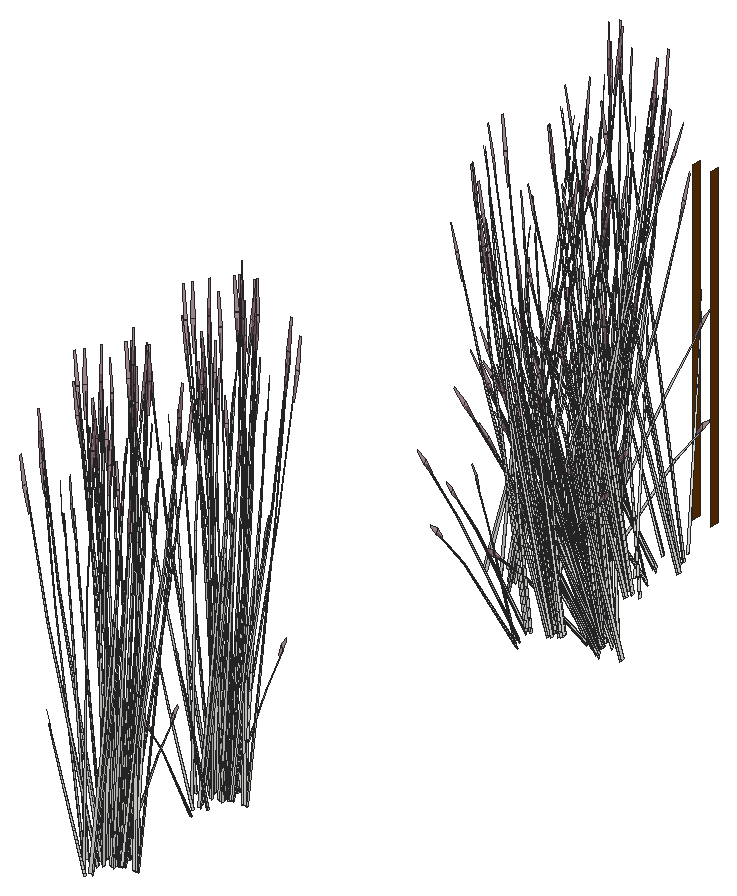
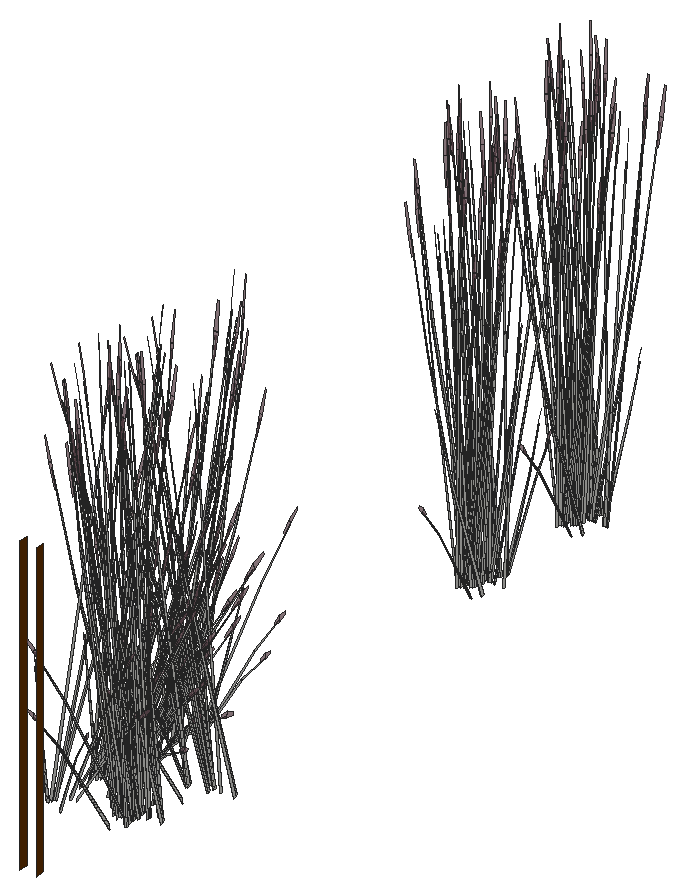
# SketchUp Ruby script. Lengths in inches.
U = 1.inch
M = Sketchup.active_model
def pt(a) = Geom::Point3d.new(a.map { |v| v * U })
def face(e, loops, mat)
  f = e.add_face(loops[0].map { |a| pt(a) })
  loops[1..].each { |l| e.add_face(l.map { |a| pt(a) }).erase! }
  f.material = f.back_material = mat if mat
  f
end
# faces: each face lists its corners as indices into pts; further lists are holes
def faces(e, pts, list, mat = nil) = list.each { |f| face(e, (f[0].is_a?(Array) ? f : [f]).map { |l| l.map { |i| pts[i] } }, mat) }
# xy, xz, yz: faces in a plane at the given z, y or x. An outline is a flat list of corners, or four numbers for a rectangle; further outlines are holes
def ring(l) = l.size == 4 ? [[l[0], l[1]], [l[2], l[1]], [l[2], l[3]], [l[0], l[3]]] : l.each_slice(2).to_a
def flat(e, list, mat, &to3) = list.each { |f| face(e, (f[0].is_a?(Array) ? f : [f]).map { |l| ring(l).map { |u, v| to3.(u, v) } }, mat) }
def xy(e, z, list, mat = nil) = flat(e, list, mat) { |x, y| [x, y, z] }
def xz(e, y, list, mat = nil) = flat(e, list, mat) { |x, z| [x, y, z] }
def yz(e, x, list, mat = nil) = flat(e, list, mat) { |y, z| [x, y, z] }
def lines(e, pts, list) = list.each { |a, b| e.add_line(pt(pts[a]), pt(pts[b])) }
# prism: a flat outline (further loops are holes) pulled along v
def prism(e, loops, v, mat = nil)
  f = face(e, loops, mat); d = Geom::Vector3d.new(v.map { |x| x * U })
  f.pushpull(f.normal.samedirection?(d) ? d.length : -d.length)
end
def box(e, o, s, mat = nil) = prism(e, [[o, [o[0] + s[0], o[1], o[2]], [o[0] + s[0], o[1] + s[1], o[2]], [o[0], o[1] + s[1], o[2]]]], [0, 0, s[2]], mat)
def at(x, y, z, deg = 0) = Geom::Transformation.translation(pt([x, y, z])) * Geom::Transformation.rotation(ORIGIN, Z_AXIS, deg.degrees)
def axes(o, x, y, z) = Geom::Transformation.new([*x, 0, *y, 0, *z, 0, *pt(o).to_a, 1])
def part(name) = M.definitions.add(name)
# library, detail: a bought-in or finely detailed component or shape, given as its bounding box
def library(name, o, s) = part(name).tap { |d| box(d.entities, o, s) }
def detail(e, o, s) = box(e.add_group.entities, o, s)
def put(e, d, t, mat = nil) = e.add_instance(d, t).tap { |i| i.material = mat if mat }
def group(e, t, mat = nil) = e.add_group.tap { |g| g.transformation = t; g.material = mat if mat }.entities
root = M.entities
M.materials.add("C08_Toffee_Ember").color = [102, 51, 0]
M.materials.add("LightPink_Translucent").color = [144, 107, 117]
M.materials["LightPink_Translucent"].alpha = 0.75
c1 = part("blade")
p = [[2.15,0.21,22],[0,0.17,0],[0.09,0.45,0],[2.18,0.31,22],[2.29,0.31,22],[0.38,0.45,0],
  [2.48,0.24,33],[2.49,0.24,33],[2.48,0.22,33]]
faces(c1.entities,p,[[0,1,2,3],[4,5,2,3],[6,3,4,7],[8,0,3,6]])
c2 = part("seeds")
p = [[0.3,-0.1,1.38],[-0.01,-0.03,1.59],[-0.01,-0.03,0.03],[0.14,-0.07,-0.07],[0.29,-0.03,3],[0.15,0.01,3.11]]
faces(c2.entities,p,[[0,1,2,3],[1,0,4,5]],"LightPink_Translucent")
c3 = part("blade with seeds")
put(c3.entities,c1,at(0,0,0))
put(c3.entities,c2,axes([2.4,0.25,30.99],[1.5799,-0.05474,1.17369],[-0.12525,1.92788,0.29478],[-0.07173,-0.02425,1.56792]))
yz(root,671.22,[[360,510,361,546]],"C08_Toffee_Ember")
yz(root,673.24,[[360,510,361,546]],"C08_Toffee_Ember")
put(root,c3,axes([670.66,276.35,511.74],[-0.26718,-0.5855,-0.57963],[0.76964,-0.21087,-0.15213],[-0.02953,-0.19827,1.27944]))
put(root,c3,axes([670.56,274.67,511.97],[-0.40676,-0.57214,0],[0.68052,-0.31907,-0.42834],[0.15499,-0.07267,1.3588]))
put(root,c3,axes([671.45,273.98,511.77],[-0.44958,0.32756,-0.03231],[-0.41194,-0.35875,-0.14649],[-0.029,-0.10165,0.48318]))
put(root,c3,axes([669.09,276.27,511.67],[0,-0.57097,-0.4121],[0.72788,0,0],[0,-0.13004,1.30728]))
put(root,c3,axes([671.11,274.58,511.67],[0.60889,-0.28548,-0.4121],[0.36394,0.51192,0],[0.13868,-0.06502,1.30728]))
put(root,c3,axes([671.07,276.5,511.83],[0.31565,-0.51449,-0.37133],[0.65588,0.24761,0.17871],[0,-0.1186,1.19224]))
put(root,c3,axes([671.36,276.25,512.21],[-0.07581,-0.65151,-0.24149],[0.7896,-0.03939,-0.41502],[0.13904,-0.08678,1.32557]))
put(root,c3,axes([669.4,276.28,511.68],[0.45414,-0.35624,-0.25712],[0.45414,0.35624,0.25712],[0,-0.11474,1.15348]))
put(root,c3,axes([670.99,276.93,512.21],[-0.73268,-0.27244,-0.24149],[0.35279,-0.57501,-0.41502],[-0.02303,-0.14118,1.32557]))
put(root,c3,axes([671.25,274.8,511.68],[0.60696,0.14127,-0.25712],[-0.15283,0.49751,0.25712],[0.12236,-0.05737,1.15348]))
put(root,c3,axes([671.46,276.76,512.02],[0.73304,0.27674,0.19974],[-0.35279,0.57501,0.41502],[0,-0.13255,1.3325]))
put(root,c3,axes([671.2,276.58,511.96],[0.28286,0.63846,0.37976],[-0.80821,0.22202,0.14902],[0.00988,-0.11732,1.31851]))
put(root,c3,axes([672.22,276.64,511.83],[0,-0.66065,0],[0.81352,0,0],[0,0,1.48949]))
put(root,c3,axes([671.83,276.22,511.96],[-0.53943,0.51816,0.37976],[-0.64086,-0.4574,0.14902],[0.13005,-0.05171,1.31851]))
put(root,c3,axes([672.42,277.15,511.91],[-0.60515,-0.49144,-0.05089],[0.60552,-0.49174,0],[-0.02113,-0.01716,1.45724]))
put(root,c3,axes([671.27,277.21,511.96],[0.82229,0.1203,0.37976],[-0.16734,0.67942,0.14902],[-0.12017,-0.06561,1.31851]))
put(root,c3,axes([672.77,276.78,511.83],[0.72788,0,0],[0,0.59111,0],[0,0,1.48078]))
put(root,c3,axes([672.53,276.48,511.98],[-0.82229,-0.1203,0.40835],[0.16734,-0.67942,0.16024],[0.12017,0.06561,1.41775]))
put(root,c3,axes([671.88,278.16,511.83],[-0.21227,-0.49226,0],[0.60616,-0.17239,0],[0,0,1.28128]))
put(root,c3,axes([672.75,277.04,511.84],[0.45414,0.3688,0],[-0.45414,0.3688,0],[0,0,1.40491]))
put(root,c3,axes([671.73,278.38,511.82],[-0.65588,-0.25634,0],[0.31565,-0.53263,0],[0,0,1.35047]))
put(root,c3,axes([672.625,276.9,511.9],[0,0.66033,-0.04679],[-0.81352,0,0],[0,0.02075,1.48875]))
put(root,c3,axes([673.02,276.72,512.17],[0.60616,-0.16651,0.12018],[0.21227,0.47548,-0.34318],[0,0.10465,1.05198]))
put(root,c3,axes([672.47,278.39,511.83],[0.65588,0.25634,0],[-0.31565,0.53263,0],[0,0,1.45212]))
put(root,c3,axes([672.73,278.96,511.82],[-0.40169,-0.57414,-0.04268],[0.68052,-0.31907,0.42834],[-0.16769,0.05466,1.35813]))
put(root,c3,axes([672.59,277.57,512.17],[0.48065,0.34305,0.12018],[-0.40092,0.38703,-0.34318],[-0.1116,0.05232,1.05198]))
put(root,c3,axes([672.24,278.18,511.9],[0.28286,0.65594,-0.0499],[-0.80821,0.22985,0],[0.00988,0.02291,1.42904]))
put(root,c3,axes([672.55,278.89,511.68],[-0.60696,-0.14127,-0.25712],[0.15283,-0.49751,0.25712],[-0.12236,0.05737,1.15348]))
put(root,c3,axes([674.57,277.32,511.83],[-0.81312,-0.00457,-0.0413],[0,-0.63814,0.41452],[-0.02555,0.14527,1.31432]))
put(root,c3,axes([672.8125,276.76,512.21],[0.73268,0.27244,-0.24149],[-0.35279,0.57501,-0.41502],[0.02303,0.14118,1.32557]))
put(root,c3,axes([674.4,277.41,511.68],[-0.45414,0.35624,-0.25712],[-0.45414,-0.35624,0.25712],[0,0.11474,1.15348]))
put(root,c3,axes([672.45,277.44,512.21],[0.07581,0.65151,-0.24149],[-0.7896,0.03939,-0.41502],[-0.13904,0.08678,1.32557]))
put(root,c3,axes([672.73,277.19,511.83],[-0.31565,0.51449,-0.37133],[-0.65588,-0.24761,0.17871],[0,0.1186,1.19224]))
put(root,c3,axes([672.75,278.67,511.93],[0.81449,0.18558,0.25528],[-0.20377,0.66335,-0.30288],[-0.13481,0.08302,1.36855]))
put(root,c3,axes([674.72,277.42,511.67],[0,0.57097,-0.4121],[-0.72788,0,0],[0,0.13004,1.30728]))
put(root,c3,axes([673.25,279.02,511.97],[0.40676,0.57214,0],[-0.68052,0.31907,-0.42834],[-0.15499,0.07267,1.3588]))
put(root,c3,axes([673.11,277.35,511.74],[0.23855,0.52277,-0.57446],[-0.68718,0.18827,-0.15077],[0.02637,0.17702,1.26801]))
put(root,c3,axes([671.11,279.2,511.24],[0.10529,-0.03107,1.46364],[0.63335,0.17101,-0.2236],[0.01852,0.19274,0.24931]))
put(root,c3,axes([669.65,279.28,512.34],[0.59102,-0.10111,0.05401],[0.13587,0.40735,-0.71633],[-0.03747,0.2062,0.64209]))
put(root,c3,axes([672.94,289.54,512.15],[-0.18493,0.11557,1.18691],[-0.55384,-0.20228,-0.25526],[0.10266,-0.25157,0.50747]))
put(root,c3,axes([671.5625,288.91,511.24],[-0.10912,0.02057,1.46364],[-0.60346,-0.23156,-0.2236],[0.01013,-0.19315,0.24931]))
put(root,c3,axes([670.66,291.68,511.74],[-0.26718,-0.5855,-0.57963],[0.76964,-0.21087,-0.15213],[-0.02953,-0.19827,1.27944]))
put(root,c3,axes([670.56,290,511.97],[-0.40676,-0.57214,0],[0.68052,-0.31907,-0.42834],[0.15499,-0.07267,1.3588]))
put(root,c3,axes([671.45,289.3125,511.77],[-0.44958,0.32756,-0.03231],[-0.41194,-0.35875,-0.14649],[-0.029,-0.10165,0.48318]))
put(root,c3,axes([671.11,289.91,511.67],[0.60889,-0.28548,-0.4121],[0.36394,0.51192,0],[0.13868,-0.06502,1.30728]))
put(root,c3,axes([671.07,291.84,511.83],[0.31565,-0.51449,-0.37133],[0.65588,0.24761,0.17871],[0,-0.1186,1.19224]))
put(root,c3,axes([671.36,291.58,512.21],[-0.07581,-0.65151,-0.24149],[0.7896,-0.03939,-0.41502],[0.13904,-0.08678,1.32557]))
put(root,c3,axes([669.4,291.62,511.68],[0.45414,-0.35624,-0.25712],[0.45414,0.35624,0.25712],[0,-0.11474,1.15348]))
put(root,c3,axes([670.99,292.26,512.21],[-0.73268,-0.27244,-0.24149],[0.35279,-0.57501,-0.41502],[-0.02303,-0.14118,1.32557]))
put(root,c3,axes([671.25,290.14,511.68],[0.60696,0.14127,-0.25712],[-0.15283,0.49751,0.25712],[0.12236,-0.05737,1.15348]))
put(root,c3,axes([671.46,292.09,512.02],[0.73304,0.27674,0.19974],[-0.35279,0.57501,0.41502],[0,-0.13255,1.3325]))
put(root,c3,axes([671.2,291.92,511.96],[0.28286,0.63846,0.37976],[-0.80821,0.22202,0.14902],[0.00988,-0.11732,1.31851]))
put(root,c3,axes([672.22,291.97,511.83],[0,-0.66065,0],[0.81352,0,0],[0,0,1.48949]))
put(root,c3,axes([671.83,291.55,511.96],[-0.53943,0.51816,0.37976],[-0.64086,-0.4574,0.14902],[0.13005,-0.05171,1.31851]))
put(root,c3,axes([672.42,292.48,511.91],[-0.60515,-0.49144,-0.05089],[0.60552,-0.49174,0],[-0.02113,-0.01716,1.45724]))
put(root,c3,axes([671.27,292.54,511.96],[0.82229,0.1203,0.37976],[-0.16734,0.67942,0.14902],[-0.12017,-0.06561,1.31851]))
put(root,c3,axes([672.77,292.12,511.83],[0.72788,0,0],[0,0.59111,0],[0,0,1.48078]))
put(root,c3,axes([672.53,291.82,511.98],[-0.82229,-0.1203,0.40835],[0.16734,-0.67942,0.16024],[0.12017,0.06561,1.41775]))
put(root,c3,axes([671.88,293.49,511.83],[-0.21227,-0.49226,0],[0.60616,-0.17239,0],[0,0,1.28128]))
put(root,c3,axes([672.75,292.37,511.84],[0.45414,0.3688,0],[-0.45414,0.3688,0],[0,0,1.40491]))
put(root,c3,axes([671.73,293.72,511.82],[-0.65588,-0.25634,0],[0.31565,-0.53263,0],[0,0,1.35047]))
put(root,c3,axes([672.625,292.23,511.9],[0,0.66033,-0.04679],[-0.81352,0,0],[0,0.02075,1.48875]))
put(root,c3,axes([673.02,292.06,512.17],[0.60616,-0.16651,0.12018],[0.21227,0.47548,-0.34318],[0,0.10465,1.05198]))
put(root,c3,axes([672.47,293.73,511.83],[0.65588,0.25634,0],[-0.31565,0.53263,0],[0,0,1.45212]))
put(root,c3,axes([672.73,294.29,511.82],[-0.40169,-0.57414,-0.04268],[0.68052,-0.31907,0.42834],[-0.16769,0.05466,1.35813]))
put(root,c3,axes([672.59,292.91,512.17],[0.48065,0.34305,0.12018],[-0.40092,0.38703,-0.34318],[-0.1116,0.05232,1.05198]))
put(root,c3,axes([672.24,293.51,511.9],[0.28286,0.65594,-0.0499],[-0.80821,0.22985,0],[0.00988,0.02291,1.42904]))
put(root,c3,axes([672.55,294.22,511.68],[-0.60696,-0.14127,-0.25712],[0.15283,-0.49751,0.25712],[-0.12236,0.05737,1.15348]))
put(root,c3,axes([674.57,292.65,511.83],[-0.81312,-0.00457,-0.0413],[0,-0.63814,0.41452],[-0.02555,0.14527,1.31432]))
put(root,c3,axes([672.8125,292.1,512.21],[0.73268,0.27244,-0.24149],[-0.35279,0.57501,-0.41502],[0.02303,0.14118,1.32557]))
put(root,c3,axes([674.4,292.74,511.68],[-0.45414,0.35624,-0.25712],[-0.45414,-0.35624,0.25712],[0,0.11474,1.15348]))
put(root,c3,axes([672.45,292.78,512.21],[0.07581,0.65151,-0.24149],[-0.7896,0.03939,-0.41502],[-0.13904,0.08678,1.32557]))
put(root,c3,axes([672.73,292.52,511.83],[-0.31565,0.51449,-0.37133],[-0.65588,-0.24761,0.17871],[0,0.1186,1.19224]))
put(root,c3,axes([672.75,294,511.93],[0.81449,0.18558,0.25528],[-0.20377,0.66335,-0.30288],[-0.13481,0.08302,1.36855]))
put(root,c3,axes([674.72,292.76,511.67],[0,0.57097,-0.4121],[-0.72788,0,0],[0,0.13004,1.30728]))
put(root,c3,axes([673.25,294.36,511.97],[0.40676,0.57214,0],[-0.68052,0.31907,-0.42834],[-0.15499,0.07267,1.3588]))
put(root,c3,axes([673.11,292.68,511.74],[0.23855,0.52277,-0.57446],[-0.68718,0.18827,-0.15077],[0.02637,0.17702,1.26801]))
put(root,c3,axes([671.11,294.53,511.24],[0.10529,-0.03107,1.46364],[0.63335,0.17101,-0.2236],[0.01852,0.19274,0.24931]))
put(root,c3,axes([669.65,294.61,512.34],[0.59102,-0.10111,0.05401],[0.13587,0.40735,-0.71633],[-0.03747,0.2062,0.64209]))
put(root,c3,axes([675.52,330.24,512.15],[-0.0394,0.18678,1.18691],[-0.57594,0.15636,-0.25526],[-0.13463,-0.24142,0.50747]))
put(root,c3,axes([675.06,330.53,511.24],[-0.06302,0.07522,1.46364],[-0.63686,0.16217,-0.2236],[-0.15385,-0.14752,0.24931]))
put(root,c3,axes([674.66,330.82,511.77],[-0.18768,0.46622,-0.03231],[-0.57763,-0.14342,-0.14649],[-0.0877,-0.07626,0.48318]))
put(root,c3,axes([674.35,332.95,511.97],[-0.81352,0,0],[0,-0.63814,-0.42834],[0,-0.14534,1.3588]))
put(root,c3,axes([674.98,332.78,511.93],[-0.60515,0.48003,0.25528],[-0.60552,-0.47498,-0.30288],[-0.02113,-0.13632,1.36855]))
put(root,c3,axes([676.62,333.78,512.02],[0.17244,-0.67657,-0.19446],[0.81759,0.11793,0.42555],[-0.14286,-0.09343,1.29846]))
put(root,c3,axes([676.5625,333.51,511.83],[-0.39083,-0.47924,-0.37133],[0.59199,-0.33747,0.17871],[-0.12647,-0.0593,1.19224]))
put(root,c3,axes([676.21,333.69,511.71],[-0.67676,-0.09361,-0.51753],[0.14281,-0.57742,-0.13583],[-0.20196,-0.06997,1.14236]))
put(root,c3,axes([674.04,332.875,511.24],[0.0165,0.08998,1.46364],[-0.33262,0.46992,-0.2236],[-0.23626,-0.02369,0.24931]))
put(root,c3,axes([675.49,334.57,511.68],[-0.15283,-0.49751,-0.25712],[0.60696,-0.14127,0.25712],[-0.12236,-0.05737,1.15348]))
put(root,c3,axes([675.32,334.79,511.67],[-0.60889,-0.28548,-0.4121],[0.36394,-0.51192,0],[-0.13868,-0.06502,1.30728]))
put(root,c3,axes([676.98,333.78,512.21],[-0.65687,0.37907,-0.24149],[-0.43681,-0.53562,-0.41502],[-0.16207,-0.0544,1.32557]))
put(root,c3,axes([676.92,333.94,512.17],[-0.12551,0.50956,0.12018],[-0.6132,-0.08845,-0.34318],[-0.1116,-0.05232,1.05198]))
put(root,c3,axes([677.72,333.95,512.05],[-0.63528,-0.45956,-0.20909],[0.53456,-0.51604,0.45758],[-0.17107,0.05376,1.39619]))
put(root,c3,axes([678.81,338.02,509.56],[-0.55475,-0.27598,-0.58968],[0.39425,-0.48361,0.07116],[-0.20099,-0.16478,0.83415]))
put(root,c3,axes([675.69,335.13,511.97],[-0.40676,0.57214,0],[-0.68052,-0.31907,-0.42834],[-0.15499,-0.07267,1.3588]))
put(root,c3,axes([677.4,333.85,511.83],[-0.70648,0.03525,-0.37133],[-0.06389,-0.58508,0.17871],[-0.12647,0.0593,1.19224]))
put(root,c3,axes([677.38,338.33,508.64],[0.24166,0.09837,1.42242],[-0.50011,0.41269,0.11501],[-0.3117,-0.18617,0.60807]))
put(root,c3,axes([678.55,338.04,509.31],[-0.64198,0.13573,-0.42412],[-0.1123,-0.514,-0.32852],[-0.17243,-0.1473,0.81151]))
put(root,c3,axes([679,337.58,509.93],[-0.4342,0.54737,-0.11304],[-0.6288,-0.31535,-0.62743],[-0.21858,-0.15465,0.95337]))
put(root,c3,axes([668.05,338.27,511.24],[-0.09738,-0.04498,1.46364],[-0.25012,-0.50252,-0.2236],[0.16873,-0.13637,0.24931]))
put(root,c3,axes([676.51,339.91,512.15],[-0.0394,0.18678,1.18691],[-0.57594,0.15636,-0.25526],[-0.13463,-0.24142,0.50747]))
put(root,c3,axes([677.33,337.42,509.34],[-0.13998,-0.00403,1.45204],[-0.44565,0.40302,-0.22964],[-0.23779,-0.08235,0.11645]))
put(root,c3,axes([677.23,338.33,509.65],[0.53728,-0.42137,0.44623],[0.46337,0.44748,0.36794],[-0.25207,-0.07773,0.92337]))
put(root,c3,axes([677.42,334.19,511.71],[-0.43821,0.42916,-0.51753],[-0.54436,-0.38915,-0.13583],[-0.1756,0.10706,1.14236]))
put(root,c3,axes([677.48,338.33,509.35],[0.03276,-0.43418,0.05337],[0.49468,0.0119,0.42015],[-0.18949,-0.04543,0.64067]))
put(root,c3,axes([677.29,338.47,509.18],[-0.37017,-0.35748,-0.29394],[0.42268,-0.3384,0.37948],[-0.21476,-0.05149,0.72609]))
put(root,c3,axes([665.65,339.46,511.71],[0.43821,-0.42916,-0.51753],[0.54436,0.38915,-0.13583],[0.1756,-0.10706,1.14236]))
put(root,c3,axes([677.15,338.85,507.57],[0.12702,0.15896,1.18691],[-0.2927,0.4321,-0.25526],[-0.30054,-0.10328,0.50747]))
put(root,c3,axes([677.68,338.71,509.56],[-0.65035,-0.01375,-0.58968],[0.04368,-0.5789,0.07116],[-0.27552,-0.06109,0.83415]))
put(root,c3,axes([673.86,335.4,511.24],[0.08727,0.05704,1.46364],[0.14797,0.52853,-0.2236],[-0.19341,0.11271,0.24931]))
put(root,c3,axes([676.04,340.21,511.24],[-0.06302,0.07522,1.46364],[-0.63686,0.16217,-0.2236],[-0.15385,-0.14752,0.24931]))
put(root,c3,axes([676.8,337.76,509.33],[0.04823,0.05698,1.47228],[-0.23252,0.51221,-0.13912],[-0.23548,0.00371,0.26054]))
put(root,c3,axes([677.46,338.82,509.31],[-0.47241,0.37822,-0.42412],[-0.41372,-0.39954,-0.32852],[-0.24002,-0.05755,0.81151]))
put(root,c3,axes([677.8125,338.65,509.62],[0.37017,0.35748,0.29394],[-0.42268,0.3384,-0.37948],[-0.21476,-0.05149,0.72609]))
put(root,c3,axes([676.4,339.32,507.72],[0.41536,-0.04086,0.95334],[-0.26347,0.35999,0.70045],[-0.20525,-0.054,0.20998]))
put(root,c3,axes([677.71,338.43,509.6],[-0.03484,0.58066,-0.10093],[-0.65957,-0.01587,-0.56021],[-0.25402,-0.04034,0.85122]))
put(root,c3,axes([676.87,339.23,508.64],[0.26985,-0.01293,1.42242],[-0.17902,0.56047,0.11501],[-0.38456,-0.03467,0.60807]))
put(root,c3,axes([667.37,338.52,511.97],[0.40676,-0.57214,0],[0.68052,0.31907,-0.42834],[0.15499,0.07267,1.3588]))
put(root,c3,axes([678.875,340.73,507.13],[-0.67676,-0.09361,-0.51753],[0.14281,-0.57742,-0.13583],[-0.20196,-0.06997,1.14236]))
put(root,c3,axes([668.97,340.79,511.65],[-0.41902,0.06852,1.17514],[-0.0667,-0.54541,0.06726],[0.29348,-0.08255,0.6687]))
put(root,c3,axes([669.74,340.3,511.875],[-0.40335,-0.3651,-0.05385],[0.44175,-0.33453,-0.24415],[0.12517,-0.02355,0.8053]))
put(root,c3,axes([676.76,339.65,509.35],[0.18381,-0.5206,0.39842],[0.60429,0.17802,0.32852],[-0.23764,0.03129,0.82444]))
put(root,c3,axes([676.71,339.51,509.35],[-0.23895,-0.38931,0.05337],[0.43573,-0.19055,0.42015],[-0.19208,0.0376,0.64067]))
put(root,c3,axes([676.7,339.91,506.66],[0.0165,0.08998,1.46364],[-0.33262,0.46992,-0.2236],[-0.23626,-0.02369,0.24931]))
put(root,c3,axes([675.65,340.5,511.77],[-0.18768,0.46622,-0.03231],[-0.57763,-0.14342,-0.14649],[-0.0877,-0.07626,0.48318]))
put(root,c3,axes([675.34,342.63,511.97],[-0.81352,0,0],[0,-0.63814,-0.42834],[0,-0.14534,1.3588]))
put(root,c3,axes([664.43,339.54,511.32],[-0.64037,0.22859,1.07011],[-0.20382,-0.65589,0.4158],[0.39323,0.01091,1.21713]))
put(root,c3,axes([675.48,341.49,512.15],[0.12702,0.15896,1.18691],[-0.2927,0.4321,-0.25526],[-0.30054,-0.10328,0.50747]))
put(root,c3,axes([669.43,340.43,511.24],[-0.034,-0.08668,1.46364],[0.23582,-0.50706,-0.2236],[0.23788,-0.00729,0.24931]))
put(root,c3,axes([674.95,335.96,512.15],[0.2053,-0.09007,1.18691],[0.50689,0.27159,-0.25526],[-0.15087,0.235,0.50747]))
put(root,c3,axes([676.63,339.71,509.18],[-0.54068,-0.15928,-0.29394],[0.1577,-0.46469,0.37948],[-0.21769,0.04261,0.72609]))
put(root,c3,axes([666.09,339.875,512.21],[0.65687,-0.37907,-0.24149],[0.43681,0.53562,-0.41502],[0.16207,0.0544,1.32557]))
put(root,c3,axes([667.74,338.87,511.67],[0.60889,0.28548,-0.4121],[-0.36394,0.51192,0],[0.13868,0.06502,1.30728]))
put(root,c3,axes([675.97,342.46,511.93],[-0.60515,0.48003,0.25528],[-0.60552,-0.47498,-0.30288],[-0.02113,-0.13632,1.36855]))
put(root,c3,axes([677.2,339.66,509.62],[0.54068,0.15928,0.29394],[-0.1577,0.46469,-0.37948],[-0.21769,0.04261,0.72609]))
put(root,c3,axes([667.57,339.08,511.68],[0.15283,0.49751,-0.25712],[-0.60696,0.14127,0.25712],[0.12236,0.05737,1.15348]))
put(root,c3,axes([678.28,339.63,508.2],[0.18493,-0.0826,1.46963],[0.06377,0.5767,0.11501],[-0.40056,0.07652,0.52526]))
put(root,c3,axes([666.85,339.96,511.71],[0.67676,0.09361,-0.51753],[-0.14281,0.57742,-0.13583],[0.20196,0.06997,1.14236]))
put(root,c3,axes([676.29,340.02,509.34],[-0.10624,0.07413,1.45204],[0.00904,0.54162,-0.22964],[-0.24352,0.07044,0.11645]))
put(root,c3,axes([677,339.94,509.31],[-0.17625,0.51936,-0.42412],[-0.60429,-0.17802,-0.32852],[-0.2433,0.04762,0.81151]))
put(root,c3,axes([676.98,339.5,509.6],[0.32734,0.51701,-0.10093],[-0.58097,0.25407,-0.56021],[-0.24483,0.06821,0.85122]))
put(root,c3,axes([669.02,346.26,512.15],[-0.18493,0.11557,1.18691],[-0.55384,-0.20228,-0.25526],[0.10266,-0.25157,0.50747]))
put(root,c3,axes([677.2,343.37,511.71],[-0.67676,-0.09361,-0.51753],[0.14281,-0.57742,-0.13583],[-0.20196,-0.06997,1.14236]))
put(root,c3,axes([675.02,342.55,511.24],[0.0165,0.08998,1.46364],[-0.33262,0.46992,-0.2236],[-0.23626,-0.02369,0.24931]))
put(root,c3,axes([676.9,340.95,509.35],[-0.16135,-0.52549,0.39842],[0.63294,-0.0912,0.32852],[-0.18654,0.12359,0.82444]))
put(root,c3,axes([676.78,340.85,509.35],[-0.44663,-0.24013,0.05337],[0.26003,-0.34195,0.42015],[-0.14319,0.11055,0.64067]))
put(root,c3,axes([676.98,340.21,508.64],[0.22574,-0.12077,1.42242],[0.19004,0.55807,0.11501],[-0.35439,0.12613,0.60807]))
put(root,c3,axes([676.48,344.25,511.68],[-0.15283,-0.49751,-0.25712],[0.60696,-0.14127,0.25712],[-0.12236,-0.05737,1.15348]))
put(root,c3,axes([676.3125,344.46,511.67],[-0.60889,-0.28548,-0.4121],[0.36394,-0.51192,0],[-0.13868,-0.06502,1.30728]))
put(root,c3,axes([677.97,343.45,512.21],[-0.65687,0.37907,-0.24149],[-0.43681,-0.53562,-0.41502],[-0.16207,-0.0544,1.32557]))
put(root,c3,axes([676.28,341.16,507.57],[0.2261,0.04687,1.18691],[0.14573,0.47875,-0.25526],[-0.30712,0.08962,0.50747]))
put(root,c3,axes([675.11,340.5625,509.33],[0.08303,0.01531,1.47228],[0.25685,0.50448,-0.13912],[-0.16996,0.13241,0.26054]))
put(root,c3,axes([675.81,342.17,507.72],[0.27113,-0.25877,0.95334],[0.10699,0.40966,0.70045],[-0.19594,0.07335,0.20998]))
put(root,c3,axes([676.83,341.05,509.18],[-0.56631,0.0816,-0.29394],[-0.14954,-0.46647,0.37948],[-0.16229,0.12529,0.72609]))
put(root,c3,axes([668.72,340.7,511.97],[0.81352,0,0],[0,0.63814,-0.42834],[0,0.14534,1.3588]))
put(root,c3,axes([670.31,346.62,511.24],[-0.09738,-0.04498,1.46364],[-0.25012,-0.50252,-0.2236],[0.16873,-0.13637,0.24931]))
put(root,c3,axes([677,346.54,511.24],[-0.06302,0.07522,1.46364],[-0.63686,0.16217,-0.2236],[-0.15385,-0.14752,0.24931]))
put(root,c3,axes([676.68,344.81,511.97],[-0.40676,0.57214,0],[-0.68052,-0.31907,-0.42834],[-0.15499,-0.07267,1.3588]))
put(root,c3,axes([677.81,340.59,508.64],[0.1625,-0.17544,1.42242],[0.41029,0.47354,0.11501],[-0.28141,0.21565,0.60807]))
put(root,c3,axes([677.3,341.1,509.31],[0.16713,0.52135,-0.42412],[-0.63294,0.0912,-0.32852],[-0.18138,0.14003,0.81151]))
put(root,c3,axes([676.52,342.43,506.66],[0.08727,0.05704,1.46364],[0.14797,0.52853,-0.2236],[-0.19341,0.11271,0.24931]))
put(root,c3,axes([667.71,342.93,511.24],[0.0474,-0.08243,1.46364],[0.59674,-0.24277,-0.2236],[0.18092,0.12565,0.24931]))
put(root,c3,axes([667.1875,346.63,511.67],[0.60889,-0.28548,-0.4121],[0.36394,0.51192,0],[0.13868,-0.06502,1.30728]))
put(root,c3,axes([667.91,347.8,511.71],[0.43821,-0.42916,-0.51753],[0.54436,0.38915,-0.13583],[0.1756,-0.10706,1.14236]))
put(root,c3,axes([677.6875,341.02,508.64],[0.12114,-0.19625,1.42242],[0.50818,0.40613,0.11501],[-0.22925,0.25313,0.60807]))
put(root,c3,axes([674.6,343.8,512.15],[0.2261,0.04687,1.18691],[0.14573,0.47875,-0.25526],[-0.30712,0.08962,0.50747]))
put(root,c3,axes([676.31,342.04,509.34],[-0.01617,0.11299,1.45204],[0.45894,0.39307,-0.22964],[-0.12015,0.18588,0.11645]))
put(root,c3,axes([667.43,348.3,512.21],[-0.07581,-0.65151,-0.24149],[0.7896,-0.03939,-0.41502],[0.13904,-0.08678,1.32557]))
put(root,c3,axes([676.6,346.83,511.77],[-0.18768,0.46622,-0.03231],[-0.57763,-0.14342,-0.14649],[-0.0877,-0.07626,0.48318]))
put(root,c3,axes([667.33,346.86,511.68],[0.60696,0.14127,-0.25712],[-0.15283,0.49751,0.25712],[0.12236,-0.05737,1.15348]))
put(root,c3,axes([676.43,347.82,512.15],[0.12702,0.15896,1.18691],[-0.2927,0.4321,-0.25526],[-0.30054,-0.10328,0.50747]))
put(root,c3,axes([678.4,343.87,511.71],[-0.43821,0.42916,-0.51753],[-0.54436,-0.38915,-0.13583],[-0.1756,0.10706,1.14236]))
put(root,c3,axes([674.85,345.07,511.24],[0.08727,0.05704,1.46364],[0.14797,0.52853,-0.2236],[-0.19341,0.11271,0.24931]))
put(root,c3,axes([669.63,346.87,511.97],[0.40676,-0.57214,0],[0.68052,0.31907,-0.42834],[0.15499,0.07267,1.3588]))
put(root,c3,axes([671.99,348.64,511.875],[-0.40335,-0.3651,-0.05385],[0.44175,-0.33453,-0.24415],[0.12517,-0.02355,0.8053]))
put(root,c3,axes([667.91,348.27,511.96],[-0.53943,0.51816,0.37976],[-0.64086,-0.4574,0.14902],[0.13005,-0.05171,1.31851]))
put(root,c3,axes([678.15,349.7,511.71],[-0.67676,-0.09361,-0.51753],[0.14281,-0.57742,-0.13583],[-0.20196,-0.06997,1.14236]))
put(root,c3,axes([666.69,347.88,511.32],[-0.64037,0.22859,1.07011],[-0.20382,-0.65589,0.4158],[0.39323,0.01091,1.21713]))
put(root,c3,axes([668.41,348.05,512.17],[0.12551,-0.50956,0.12018],[0.6132,0.08845,-0.34318],[0.1116,0.05232,1.05198]))
put(root,c3,axes([675.97,348.88,511.24],[0.0165,0.08998,1.46364],[-0.33262,0.46992,-0.2236],[-0.23626,-0.02369,0.24931]))
put(root,c3,axes([668.34,348.22,512.21],[0.65687,-0.37907,-0.24149],[0.43681,0.53562,-0.41502],[0.16207,0.0544,1.32557]))
put(root,c3,axes([670,347.21,511.67],[0.60889,0.28548,-0.4121],[-0.36394,0.51192,0],[0.13868,0.06502,1.30728]))
put(root,c3,axes([668.84,348.84,511.83],[0.72788,0,0],[0,0.59111,0],[0,0,1.48078]))
put(root,c3,axes([677.26,350.79,511.67],[-0.60889,-0.28548,-0.4121],[0.36394,-0.51192,0],[-0.13868,-0.06502,1.30728]))
put(root,c3,axes([669.83,347.42,511.68],[0.15283,0.49751,-0.25712],[-0.60696,0.14127,0.25712],[0.12236,0.05737,1.15348]))
put(root,c3,axes([668.61,348.54,511.98],[-0.82229,-0.1203,0.40835],[0.16734,-0.67942,0.16024],[0.12017,0.06561,1.41775]))
put(root,c3,axes([668.75,350.15,511.8125],[0.68303,-0.19373,-0.15934],[0.24001,0.55805,0.00007],[0.07539,-0.02141,1.44335]))
put(root,c3,axes([668.83,349.09,511.84],[0.45414,0.3688,0],[-0.45414,0.3688,0],[0,0,1.40491]))
put(root,c3,axes([675.94,345.64,512.15],[0.2053,-0.09007,1.18691],[0.50689,0.27159,-0.25526],[-0.15087,0.235,0.50747]))
put(root,c3,axes([669.11,348.3,511.71],[0.67676,0.09361,-0.51753],[-0.14281,0.57742,-0.13583],[0.20196,0.06997,1.14236]))
put(root,c3,axes([668.76,348.49,511.83],[0.39083,0.47924,-0.37133],[-0.59199,0.33747,0.17871],[0.12647,0.0593,1.19224]))
put(root,c3,axes([669.1,348.78,512.17],[0.60616,-0.16651,0.12018],[0.21227,0.47548,-0.34318],[0,0.10465,1.05198]))
put(root,c3,axes([677.63,351.14,511.97],[-0.40676,0.57214,0],[-0.68052,-0.31907,-0.42834],[-0.15499,-0.07267,1.3588]))
put(root,c3,axes([668.55,350.45,511.83],[0.65588,0.25634,0],[-0.31565,0.53263,0],[0,0,1.45212]))
put(root,c3,axes([670.97,349.04,511.97],[0.81352,0,0],[0,0.63814,-0.42834],[0,0.14534,1.3588]))
put(root,c3,axes([668.89,348.82,512.21],[0.73268,0.27244,-0.24149],[-0.35279,0.57501,-0.41502],[0.02303,0.14118,1.32557]))
put(root,c3,axes([675.55,350.14,512.15],[0.2261,0.04687,1.18691],[0.14573,0.47875,-0.25526],[-0.30712,0.08962,0.50747]))
put(root,c3,axes([670.48,349.47,511.68],[-0.45414,0.35624,-0.25712],[-0.45414,-0.35624,0.25712],[0,0.11474,1.15348]))
put(root,c3,axes([670.79,349.48,511.67],[0,0.57097,-0.4121],[-0.72788,0,0],[0,0.13004,1.30728]))
put(root,c3,axes([669.97,351.27,511.24],[0.0474,-0.08243,1.46364],[0.59674,-0.24277,-0.2236],[0.18092,0.12565,0.24931]))
put(root,c3,axes([669.18,349.4,511.74],[0.23855,0.52277,-0.57446],[-0.68718,0.18827,-0.15077],[0.02637,0.17702,1.26801]))
put(root,c3,axes([675.8,351.41,511.24],[0.08727,0.05704,1.46364],[0.14797,0.52853,-0.2236],[-0.19341,0.11271,0.24931]))
put(root,c3,axes([668.5625,350.49,512.15],[0.01148,-0.18927,1.18691],[0.54864,-0.21141,-0.25526],[0.16937,0.22654,0.50747]))
put(root,c3,axes([676.89,351.97,512.15],[0.2053,-0.09007,1.18691],[0.50689,0.27159,-0.25526],[-0.15087,0.235,0.50747]))
